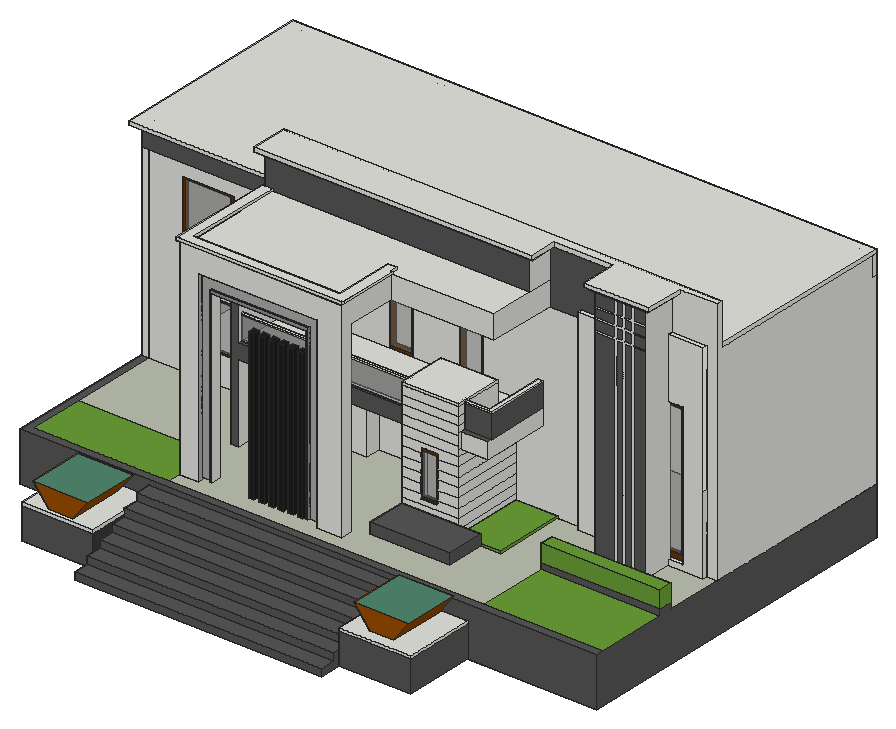
# SketchUp Ruby script. Lengths in inches.
U = 1.inch
M = Sketchup.active_model
def pt(a) = Geom::Point3d.new(a.map { |v| v * U })
def face(e, loops, mat)
  f = e.add_face(loops[0].map { |a| pt(a) })
  loops[1..].each { |l| e.add_face(l.map { |a| pt(a) }).erase! }
  f.material = f.back_material = mat if mat
  f
end
# faces: each face lists its corners as indices into pts; further lists are holes
def faces(e, pts, list, mat = nil) = list.each { |f| face(e, (f[0].is_a?(Array) ? f : [f]).map { |l| l.map { |i| pts[i] } }, mat) }
# xy, xz, yz: faces in a plane at the given z, y or x. An outline is a flat list of corners, or four numbers for a rectangle; further outlines are holes
def ring(l) = l.size == 4 ? [[l[0], l[1]], [l[2], l[1]], [l[2], l[3]], [l[0], l[3]]] : l.each_slice(2).to_a
def flat(e, list, mat, &to3) = list.each { |f| face(e, (f[0].is_a?(Array) ? f : [f]).map { |l| ring(l).map { |u, v| to3.(u, v) } }, mat) }
def xy(e, z, list, mat = nil) = flat(e, list, mat) { |x, y| [x, y, z] }
def xz(e, y, list, mat = nil) = flat(e, list, mat) { |x, z| [x, y, z] }
def yz(e, x, list, mat = nil) = flat(e, list, mat) { |y, z| [x, y, z] }
def lines(e, pts, list) = list.each { |a, b| e.add_line(pt(pts[a]), pt(pts[b])) }
# prism: a flat outline (further loops are holes) pulled along v
def prism(e, loops, v, mat = nil)
  f = face(e, loops, mat); d = Geom::Vector3d.new(v.map { |x| x * U })
  f.pushpull(f.normal.samedirection?(d) ? d.length : -d.length)
end
def box(e, o, s, mat = nil) = prism(e, [[o, [o[0] + s[0], o[1], o[2]], [o[0] + s[0], o[1] + s[1], o[2]], [o[0], o[1] + s[1], o[2]]]], [0, 0, s[2]], mat)
def at(x, y, z, deg = 0) = Geom::Transformation.translation(pt([x, y, z])) * Geom::Transformation.rotation(ORIGIN, Z_AXIS, deg.degrees)
def axes(o, x, y, z) = Geom::Transformation.new([*x, 0, *y, 0, *z, 0, *pt(o).to_a, 1])
def part(name) = M.definitions.add(name)
# library, detail: a bought-in or finely detailed component or shape, given as its bounding box
def library(name, o, s) = part(name).tap { |d| box(d.entities, o, s) }
def detail(e, o, s) = box(e.add_group.entities, o, s)
def put(e, d, t, mat = nil) = e.add_instance(d, t).tap { |i| i.material = mat if mat }
def group(e, t, mat = nil) = e.add_group.tap { |g| g.transformation = t; g.material = mat if mat }.entities
root = M.entities
M.materials.add("[Color C07]").color = [153, 76, 0]
M.materials.add("[Color C08]").color = [102, 51, 0]
M.materials.add("[Color M00]").color = [255, 255, 255]
M.materials.add("[Color M03]").color = [170, 170, 170]
M.materials.add("[Color M04]").color = [142, 142, 142]
M.materials.add("[Color M06]").color = [86, 86, 86]
M.materials.add("[Color M07]").color = [58, 58, 58]
M.materials.add("[Color M08]").color = [30, 30, 30]
M.materials.add("[Grass Dark Green]").color = [106, 157, 55]
M.materials.add("[Metal Seamed]").color = [118, 119, 115]
M.materials.add("[Pavers with Grass Brick]").color = [187, 192, 176]
M.materials.add("[Stone Vein Gray]").color = [166, 165, 165]
M.materials.add("[Translucent Glass Gray]").color = [128, 128, 128]
M.materials["[Translucent Glass Gray]"].alpha = 0.5
M.materials.add("[Vegetation Ivy Hedera]").color = [81, 134, 109]
M.materials.add("[Wood Veneer 01]").color = [120, 70, 37]
c1 = part("Group\#1")
xy(c1.entities,0,[[0,0,111.125,4.8125]])
xy(c1.entities,6.26,[[6.26,0,36.94,4.8125],[36.94,0,39.92,4.8125],[39.92,0,72.69,4.8125],[72.69,0,75.67,4.8125],[75.67,0,104.87,4.8125]],"[Color C08]")
xy(c1.entities,151.68,[[6.26,0,104.87,4.8125]],"[Color C08]")
xy(c1.entities,157.9375,[[0,0,111.125,4.8125]],"[Color C08]")
xz(c1.entities,0,[[[0,0,111.125,157.9375],[6.26,6.26,104.87,151.68]]],"[Color C08]")
xz(c1.entities,0,[[6.26,6.26,104.87,151.68]],"[Translucent Glass Gray]")
xz(c1.entities,4.8125,[[[0,0,111.125,157.9375],[6.26,6.26,104.87,151.68]]],"[Color C08]")
yz(c1.entities,0,[[0,0,4.8125,157.9375]],"[Color C08]")
yz(c1.entities,6.26,[[0,6.26,4.8125,151.68]],"[Color C08]")
yz(c1.entities,104.87,[[0,6.26,4.8125,151.68]],"[Color C08]")
yz(c1.entities,111.125,[[0,0,4.8125,157.9375]],"[Color C08]")
xy(root,-66.5625,[[11,144,11,684,900.0625,684,900.0625,144,209.9,144,209.9,145.85,99.84,145.85,99.84,144]])
xy(root,-66.5625,[[590.88,33.9375,700.95,144],[99.84,35.78,209.9,144],[99.84,144,209.9,145.85]],"[Color M06]")
xy(root,-18.5625,[[590.88,33.9375,700.95,144],[99.84,35.78,209.9,145.85]])
xy(root,-13.5625,[[[590.88,33.9375,700.95,144],[624.02,51.36,662.08,138.36]],[99.84,35.78,209.9,145.85],[624.02,51.36,662.08,138.36]])
xy(root,-9.6875,[[139.78,37.5,177.84,124.49]])
xy(root,6.25,[[719,386.8125,883.625,672]])
xy(root,9,[[501.4375,266.5625,589.01,342.0625],[589.01,266.5625,654.375,377.5625],[231.74,274.5625,231.74,351.0625,243.375,351.0625,243.375,386.8125,380.41,386.8125,380.41,351.0625,243.375,351.0625,243.375,274.5625],[501.4375,342.0625,501.4375,351.0625,478.41,351.0625,478.41,386.8125,883.625,386.8125,883.625,370.25,829.89,370.25,829.89,373.5,750.2,373.5,750.2,370.25,690.45,370.25,690.45,377.5625,589.01,377.5625,589.01,342.0625],[750.2,370.25,829.89,373.5],
  [11,377.5625,11,684,900.0625,684,900.0625,377.5625,883.625,377.5625,883.625,672,23,672,23,377.5625],[23,377.5625,231.74,386.8125],[23,386.8125,231.74,672]])
xy(root,9,[[11,144,900.0625,144,900.0625,156,23,156,23,377.5625,11,377.5625]],"[Color M06]")
xy(root,9,[[23,156,230.83,241.11],[716.24,156,900.0625,266.78]],"[Grass Dark Green]")
xy(root,9,[[[230.83,156,716.24,156,716.24,287.99,900.0625,287.99,900.0625,377.5625,883.625,377.5625,883.625,370.25,829.89,370.25,829.89,328,750.2,328,750.2,370.25,690.45,370.25,690.45,377.5625,654.375,377.5625,654.375,266.5625,624.0625,266.5625,624.0625,206.125,501.4375,206.125,501.4375,351.0625,478.41,351.0625,478.41,374.5625,380.41,374.5625,380.41,351.0625,243.375,351.0625,243.375,274.5625,231.74,274.5625,231.74,377.5625,23,377.5625,23,241.11,230.83,241.11],[442.4,176.6875,480.58,194.92],[331.03,183.97,339.78,194.35],[346.85,183.97,355.6,194.35],[362.1,183.97,370.85,194.35],[376.91,183.97,385.66,194.35],[391.66,183.97,400.41,194.35],[406.6,183.97,415.35,194.35]]],"[Pavers with Grass Brick]")
xy(root,9,[[501.4375,206.125,624.0625,266.5625]],"[Stone Vein Gray]")
xy(root,9.3125,[[231.74,176.6875,260.125,194.92]])
xy(root,12,[[589.01,266.5625,654.375,377.5625]],"[Grass Dark Green]")
xy(root,12.375,[[274.3,180,277.43,194.92],[260.125,183.375,274.3,194.92]])
xy(root,13.5625,[[422.47,180,425.53,194.92],[425.53,183.375,442.4,194.92]])
xy(root,17.02,[[599.9375,51.36,685.27,138.36]],"[Vegetation Ivy Hedera]")
xy(root,17.15,[[716.97,370.25,760.76,370.25,760.76,373.5,810.51,373.5,810.51,370.25,852.41,370.25,852.41,386.8125,716.97,386.8125],[760.76,370.25,810.51,373.5]])
xy(root,18,[[716.24,266.78,900.0625,287.99]])
xy(root,20.89,[[115.69,37.5,201.02,124.49]],"[Vegetation Ivy Hedera]")
xy(root,25.1875,[[501.4375,206.125,624.0625,266.5625]],"[Color M06]")
xy(root,42.92,[[532.43,266.5625,556.68,275.5625]])
xy(root,45,[[716.24,266.78,900.0625,287.99]],"[Grass Dark Green]")
xy(root,51.8,[[74.49,377.5625,153.11,386.8125]])
xy(root,110.3125,[[380.41,351.0625,478.41,374.5625],[380.41,374.5625,478.41,386.8125]])
xy(root,111.85,[[532.43,266.5625,556.68,275.5625]])
xy(root,127.36,[[74.49,377.5625,153.11,386.8125]])
xy(root,129,[[589.01,270.875,631.25,377.5625],[243.375,274.5625,501.4375,351.0625],[501.4375,342.0625,589.01,377.5625],[243.375,351.0625,283.875,377.5625],[283.875,351.0625,380.41,377.5625],
  [380.41,351.0625,478.41,377.5625],[478.41,351.0625,501.4375,377.5625],[380.41,377.5625,478.41,377.5625,478.41,386.8125,883.625,386.8125,883.625,672,243.375,672,243.375,386.8125,380.41,386.8125]])
xy(root,153,[[243.375,278.6875,501.4375,283.59],[589.01,278.6875,631.25,283.59],[243.375,283.59,501.4375,283.59,501.4375,342.0625,589.01,342.0625,589.01,283.59,623.4375,283.59,623.4375,377.5625,537.88,377.5625,537.88,386.8125,501.88,386.8125,501.88,377.5625,430.25,377.5625,430.25,386.8125,394.25,386.8125,394.25,377.5625,322.66,377.5625,322.66,386.8125,274.66,386.8125,274.66,377.5625,243.375,377.5625]])
xy(root,153,[[589.01,270.875,631.25,278.6875],[243.375,274.5625,501.4375,278.6875]],"[Color M06]")
xy(root,189,[[[501.4375,266.5625,589.01,342.0625],[504.68,269.8,585.77,338.82]],[504.68,269.8,585.77,338.82],[243.375,278.6875,501.4375,283.59],[589.01,278.6875,631.25,283.59],[623.4375,283.59,631.25,377.5625]])
xy(root,191,[[243.375,278.6875,501.4375,283.59],[589.01,278.6875,631.25,278.6875,631.25,377.5625,623.4375,377.5625,623.4375,283.59,589.01,283.59]])
xy(root,193,[[501.4375,266.5625,589.01,342.0625]])
xy(root,203.11,[[74.49,377.5625,153.11,386.8125]])
xy(root,236.29,[[716.97,370.25,716.97,386.8125,852.41,386.8125,852.41,370.25,810.51,370.25,810.51,373.5,760.76,373.5,760.76,370.25],[760.76,370.25,810.51,373.5]])
xy(root,237,[[274.66,377.5625,322.66,386.8125],[394.25,377.5625,430.25,386.8125],[501.88,377.5625,537.88,386.8125]])
xy(root,238.5,[[331.03,183.97,339.78,194.35],[346.85,183.97,355.6,194.35],[362.1,183.97,370.85,194.35],[376.91,183.97,385.66,194.35],[391.66,183.97,400.41,194.35],
  [406.6,183.97,415.35,194.35]],"[Color M08]")
xy(root,246.62,[[750.2,370.25,829.89,373.5]])
xy(root,273.9375,[[277.43,180,422.47,194.92],[274.3,183.375,277.43,194.92],[422.47,183.375,425.53,194.92]])
xy(root,277.9375,[[277.43,183.375,422.47,194.92]])
xy(root,277.9375,[[274.3,180,425.53,183.375]],"[Color M04]")
xy(root,278.67,[[74.49,377.5625,153.11,386.8125]])
xy(root,293.9375,[[272.1,206.49,272.1,377.5625,615.91,377.5625,615.91,293.74,464.91,293.74,464.91,206.49,435.8,206.49,435.8,293.74,430.51,302.06,423.89,309.35,416.12,315.42,407.43,320.07,398.08,323.17,388.33,324.64,378.48,324.43,368.81,322.54,359.6,319.04,351.12,314.02,343.61,307.625,337.31,300.05,337.31,206.49]])
xy(root,297.1875,[[260.125,183.375,393.59,183.375,260.125,193.64],[393.59,183.375,442.4,183.375,442.4,194.92,260.125,194.92,260.125,193.64],[260.125,193.64,260.125,194.92,243.375,194.92],[231.74,194.92,243.375,274.5625],[243.375,194.92,243.375,377.5625,272.1,377.5625,272.1,206.49,464.91,206.49,464.91,293.74,615.91,293.74,615.91,377.5625,640.81,377.5625,640.81,270.875,480.58,270.875,480.58,194.92],
  [337.31,206.49,337.31,300.05,343.61,307.625,351.12,314.02,359.6,319.04,368.81,322.54,378.48,324.43,388.33,324.64,398.08,323.17,407.43,320.07,416.12,315.42,423.89,309.35,430.51,302.06,435.8,293.74,435.8,206.49],[243.375,377.5625,480.76,386.8125],[11,676.625,900.0625,684]])
xy(root,297.1875,[[260.125,176.6875,442.4,176.6875,442.4,179.62,393.59,183.375,260.125,183.375],[442.4,179.62,442.4,183.375,393.59,183.375]],"[Color M03]")
xy(root,309.625,[[690.45,370.25,750.2,377.5625]])
xy(root,327.1875,[[0,367.4375,0,684,11,684,11,676.625,900.0625,676.625,900.0625,386.8125,231.74,386.8125,231.74,367.4375],[11,676.625,900.0625,684]])
xy(root,328.1875,[[829.89,370.25,883.625,377.5625]])
xy(root,333.1875,[[227.99,173.625,228.81,176.6875],[228.81,173.625,231.74,176.6875],[231.74,173.625,480.58,176.6875],[480.58,173.625,483.95,176.6875],[227.99,176.6875,231.74,340.0625],
  [231.74,176.6875,231.74,340.0625,243.375,340.0625,243.375,189.17,318.2,189.17,480.58,176.6875],[480.58,176.6875,318.2,189.17,467.72,189.17,467.72,282.5,480.58,282.5],[480.58,176.6875,483.95,270.875],[243.375,189.17,318.2,189.17,243.375,194.92],[318.2,189.17,467.72,189.17,467.72,282.5,480.58,282.5,480.58,270.875,640.81,270.875,640.81,340.0625,243.375,340.0625,243.375,194.92],
  [231.74,340.0625,640.81,386.8125],[0,367.4375,231.74,367.4375,231.74,386.8125,900.0625,386.8125,900.0625,684,0,684]])
xy(root,337.1875,[[227.99,173.625,483.95,173.625,483.95,270.875,480.58,270.875,480.58,282.5,467.72,282.5,467.72,189.17,243.375,189.17,243.375,340.0625,227.99,340.0625]])
xy(root,381.1875,[[746.76,321.5,746.76,377.5625,750.2,377.5625,750.2,328,829.89,328,829.89,377.5625,836.7,377.5625,836.7,321.5],[750.2,328,829.89,377.5625],[230.37,336.3125,647.56,340.0625],[230.37,340.0625,231.74,386.8125],[640.81,340.0625,647.56,377.5625]])
xy(root,385.1875,[[741.39,318.9375,741.39,373.6875,746.76,373.6875,746.76,321.5,836.7,321.5,836.7,377.5625,841.57,377.5625,841.57,318.9375],[222.81,330.5,647.56,336.3125],[647.56,330.5,651.06,373.6875],[222.81,336.3125,230.37,386.8125],[647.56,373.6875,746.76,377.5625],
  [746.76,373.6875,750.2,377.5625]])
xy(root,391.1875,[[741.39,318.9375,841.57,318.9375,841.57,377.5625,900.0625,377.5625,900.0625,386.8125,222.81,386.8125,222.81,330.5,651.06,330.5,651.06,373.6875,741.39,373.6875]])
xz(root,33.9375,[[590.88,-18.5625,700.95,-13.5625]])
xz(root,33.9375,[[590.88,-66.5625,700.95,-18.5625]],"[Color M06]")
xz(root,35.78,[[99.84,-18.5625,209.9,-13.5625]])
xz(root,35.78,[[99.84,-66.5625,209.9,-18.5625]],"[Color M06]")
xz(root,37.5,[[139.78,-9.6875,177.84,-9.6875,201.02,20.89,115.69,20.89]],"[Color C07]")
xz(root,51.36,[[624.02,-13.5625,662.08,-13.5625,685.27,17.02,599.9375,17.02]],"[Color C07]")
xz(root,124.49,[[139.78,-9.6875,115.69,20.89,201.02,20.89,177.84,-9.6875]],"[Color C07]")
xz(root,138.36,[[624.02,-13.5625,599.9375,17.02,685.27,17.02,662.08,-13.5625]],"[Color C07]")
xz(root,144,[[590.88,-66.5625,700.95,-18.5625],[590.88,-18.5625,700.95,-13.5625]])
xz(root,144,[[11,-66.5625,590.88,-66.5625,590.88,-13.5625,700.95,-13.5625,700.95,-66.5625,900.0625,-66.5625,900.0625,9,11,9],[590.88,-18.5625,700.95,-13.5625]],"[Color M06]")
xz(root,145.85,[[99.84,-66.5625,209.9,-18.5625],[99.84,-18.5625,209.9,-13.5625]])
xz(root,173.625,[[227.99,333.1875,483.95,337.1875]])
xz(root,176.6875,[[442.4,9,480.58,9,480.58,333.1875,231.74,333.1875,231.74,9.3125,260.125,9.3125,260.125,297.1875,442.4,297.1875]])
xz(root,180,[[274.3,12.375,277.43,12.375,277.43,273.9375,422.47,273.9375,422.47,13.5625,425.53,13.5625,425.53,277.9375,274.3,277.9375]],"[Color M04]")
xz(root,183.375,[[274.3,273.9375,277.43,277.9375],[422.47,273.9375,425.53,277.9375]])
xz(root,183.375,[[260.125,12.375,274.3,12.375,274.3,277.9375,425.53,277.9375,425.53,13.5625,442.4,13.5625,442.4,297.1875,260.125,297.1875]],"[Color M03]")
xz(root,183.97,[[331.03,9,339.78,238.5],[346.85,9,355.6,238.5],[362.1,9,370.85,238.5],[376.91,9,385.66,238.5],[391.66,9,400.41,238.5],
  [406.6,9,415.35,238.5]],"[Color M08]")
xz(root,189.17,[[243.375,333.1875,467.72,337.1875]])
xz(root,194.35,[[331.03,9,339.78,238.5],[346.85,9,355.6,238.5],[362.1,9,370.85,238.5],[376.91,9,385.66,238.5],[391.66,9,400.41,238.5],
  [406.6,9,415.35,238.5]],"[Color M08]")
xz(root,194.92,[[442.4,9,480.58,297.1875],[231.74,9.3125,260.125,297.1875],[260.125,12.375,260.125,297.1875,442.4,297.1875,442.4,13.5625,425.53,13.5625,425.53,273.9375,422.47,273.9375,422.47,277.9375,277.43,277.9375,277.43,273.9375,274.3,273.9375,274.3,12.375],[274.3,12.375,277.43,273.9375],[422.47,13.5625,425.53,273.9375],
  [277.43,273.9375,422.47,277.9375]])
xz(root,206.125,[[501.4375,9,624.0625,25.1875]],"[Color M06]")
xz(root,206.49,[[272.1,293.9375,337.31,297.1875],[435.8,293.9375,464.91,297.1875]])
xz(root,266.5625,[[501.4375,9,589.01,19.37],[501.4375,19.37,589.01,25.1875],[501.4375,25.1875,589.01,33.68],[501.4375,33.68,589.01,33.68,589.01,47.99,558.02,47.99,558.02,41.57,531.09,41.57,531.09,47.99,501.4375,47.99],[[531.09,41.57,558.02,113.19],[532.43,42.92,556.68,111.85]],
  [501.4375,47.99,531.09,62.3],[558.02,47.99,589.01,62.3],[501.4375,62.3,531.09,76.62],[558.02,62.3,589.01,76.62],[501.4375,76.62,531.09,90.93],
  [558.02,76.62,589.01,90.93],[501.4375,90.93,531.09,105.24],[558.02,90.93,589.01,105.24],[501.4375,105.24,531.09,105.24,531.09,113.19,558.02,113.19,558.02,105.24,589.01,105.24,589.01,119.55,501.4375,119.55],[501.4375,119.55,589.01,133.87],
  [501.4375,133.87,589.01,148.18],[501.4375,148.18,589.01,162.49],[501.4375,162.49,589.01,174.81],[501.4375,174.81,589.01,189],[501.4375,189,589.01,193]])
xz(root,266.5625,[[589.01,9,624.0625,12],[589.01,12,624.0625,25.1875]],"[Color M06]")
xz(root,266.5625,[[624.0625,9,654.375,12]],"[Grass Dark Green]")
xz(root,266.78,[[716.24,9,900.0625,18]],"[Color M06]")
xz(root,266.78,[[716.24,18,900.0625,45]],"[Grass Dark Green]")
xz(root,270.875,[[589.01,129,631.25,153],[480.58,297.1875,640.81,333.1875],[480.58,333.1875,483.95,337.1875]])
xz(root,274.5625,[[231.74,9,243.375,9,243.375,129,501.4375,129,501.4375,153,243.375,153,243.375,297.1875,231.74,297.1875]],"[Color M06]")
xz(root,275.5625,[[532.43,42.92,556.68,111.85]])
xz(root,278.6875,[[243.375,189,501.4375,191],[589.01,189,631.25,191]])
xz(root,278.6875,[[589.01,153,631.25,189]],"[Color M06]")
xz(root,278.6875,[[243.375,153,501.4375,189]],"[Translucent Glass Gray]")
xz(root,282.5,[[467.72,333.1875,480.58,337.1875]])
xz(root,283.59,[[589.01,153,623.4375,189],[243.375,189,501.4375,191],[589.01,189,623.4375,191]])
xz(root,283.59,[[243.375,153,501.4375,189]],"[Translucent Glass Gray]")
xz(root,287.99,[[716.24,9,900.0625,18]],"[Color M06]")
xz(root,287.99,[[716.24,18,900.0625,45]],"[Grass Dark Green]")
xz(root,293.74,[[464.91,293.9375,615.91,297.1875]])
xz(root,318.9375,[[741.39,385.1875,841.57,391.1875]])
xz(root,321.5,[[746.76,381.1875,836.7,385.1875]])
xz(root,328,[[[781.13,9,784.6,9,784.6,321.8,793.32,321.8,793.32,9,796.79,9,796.79,321.8,806.82,321.8,806.82,9,810.29,9,810.29,321.8,829.89,321.8,829.89,324.21,810.29,324.21,810.29,339.86,829.89,339.86,829.89,342.27,810.29,342.27,810.29,355.8,829.89,355.8,829.89,358.21,810.29,358.21,810.29,381.1875,806.82,381.1875,806.82,358.21,796.79,358.21,796.79,381.1875,793.32,381.1875,793.32,358.21,784.6,358.21,784.6,381.1875,781.13,381.1875,781.13,358.21,750.2,358.21,750.2,355.8,781.13,355.8,781.13,342.27,750.2,342.27,750.2,339.86,781.13,339.86,781.13,324.21,750.2,324.21,750.2,321.8,781.13,321.8],[796.79,324.21,806.82,339.86],[784.6,324.21,793.32,339.86],[796.79,342.27,806.82,355.8],[784.6,342.27,793.32,355.8]]])
xz(root,328,[[750.2,9,781.13,321.8],[784.6,9,793.32,321.8],[796.79,9,806.82,321.8],[810.29,9,829.89,321.8],[750.2,324.21,781.13,339.86],
  [784.6,324.21,793.32,339.86],[796.79,324.21,806.82,339.86],[810.29,324.21,829.89,339.86],[750.2,342.27,781.13,355.8],[784.6,342.27,793.32,355.8],
  [796.79,342.27,806.82,355.8],[810.29,342.27,829.89,355.8],[750.2,358.21,781.13,381.1875],[784.6,358.21,793.32,381.1875],[796.79,358.21,806.82,381.1875],
  [810.29,358.21,829.89,381.1875]],"[Color M06]")
xz(root,330.5,[[222.81,385.1875,651.06,391.1875]])
xz(root,336.3125,[[230.37,381.1875,647.56,385.1875]])
xz(root,340.0625,[[227.99,333.1875,231.74,337.1875],[231.74,333.1875,243.375,337.1875]])
xz(root,340.0625,[[243.375,333.1875,640.81,333.1875,640.81,381.1875,231.74,381.1875,231.74,337.1875,243.375,337.1875]],"[Color M06]")
xz(root,342.0625,[[501.4375,129,589.01,153],[501.4375,153,589.01,189],[501.4375,189,589.01,193]])
xz(root,351.0625,[[243.375,9,380.41,9,380.41,110.3125,478.41,110.3125,478.41,9,501.4375,9,501.4375,129,243.375,129]])
xz(root,367.4375,[[0,327.1875,231.74,333.1875]])
xz(root,370.25,[[[690.45,9,883.625,9,883.625,328.1875,829.89,328.1875,829.89,246.62,750.2,246.62,750.2,309.625,690.45,309.625],[716.97,17.15,852.41,236.29]]])
xz(root,373.5,[[750.2,9,829.89,17.15],[750.2,17.15,829.89,236.29],[750.2,236.29,829.89,246.62]])
xz(root,373.6875,[[651.06,385.1875,741.39,391.1875]])
xz(root,374.5625,[[380.41,9,478.41,110.3125]])
xz(root,377.5625,[[11,9,23,297.1875],[[23,9,231.74,297.1875],[74.49,203.11,153.11,278.67],[74.49,51.8,153.11,127.36]],[654.375,9,690.45,9,690.45,297.1875,615.91,297.1875,615.91,293.9375,272.1,293.9375,272.1,297.1875,243.375,297.1875,243.375,153,274.66,153,274.66,237,322.66,237,322.66,153,394.25,153,394.25,237,430.25,237,430.25,153,501.88,153,501.88,237,537.88,237,537.88,153,623.4375,153,623.4375,191,631.25,191,631.25,129,589.01,129,589.01,12,654.375,12],[589.01,9,654.375,12],[883.625,9,900.0625,9,900.0625,391.1875,841.57,391.1875,841.57,385.1875,836.7,385.1875,836.7,381.1875,829.89,381.1875,829.89,328.1875,883.625,328.1875],
  [272.1,293.9375,480.76,297.1875],[750.2,297.1875,829.89,381.1875]])
xz(root,377.5625,[[11,297.1875,231.74,327.82],[640.81,297.1875,690.45,297.1875,690.45,309.625,750.2,309.625,750.2,381.1875,746.76,381.1875,746.76,385.1875,647.56,385.1875,647.56,381.1875,640.81,381.1875]],"[Color M06]")
xz(root,386.8125,[[243.375,9,380.41,129],[478.41,9,478.41,129,716.97,129,716.97,17.15,719,17.15,719,9],[719,9,719,17.15,852.41,17.15,852.41,129,883.625,129,883.625,9],[716.97,17.15,719,129],[719,17.15,852.41,129],
  [[380.41,110.3125,380.41,129,243.375,129,243.375,297.1875,883.625,297.1875,883.625,129,852.41,129,852.41,236.29,716.97,236.29,716.97,129,478.41,129,478.41,110.3125],[274.66,153,322.66,237],[394.25,153,430.25,237],[501.88,153,537.88,237]],[243.375,297.1875,883.625,327.1875],[231.74,327.1875,243.375,333.1875],[243.375,327.1875,640.81,333.1875],[640.81,327.1875,883.625,333.1875],
  [883.625,327.1875,900.0625,333.1875],[231.74,333.1875,243.375,381.1875],[243.375,333.1875,640.81,381.1875],[640.81,333.1875,900.0625,391.1875],[230.37,381.1875,243.375,385.1875],
  [243.375,381.1875,640.81,385.1875],[222.81,385.1875,243.375,391.1875],[243.375,385.1875,640.81,391.1875]])
xz(root,672,[[719,6.25,883.625,9],[23,9,231.74,297.1875],[231.74,9,243.375,129],[243.375,9,719,129],[719,9,883.625,129],
  [231.74,129,243.375,297.1875],[243.375,129,883.625,297.1875]])
xz(root,684,[[11,9,900.0625,297.1875],[11,297.1875,900.0625,327.1875],[0,327.1875,11,327.82],[11,327.1875,11,327.82,0,327.82,0,333.1875,900.0625,333.1875,900.0625,327.1875]])
xz(root,684,[[11,-66.5625,900.0625,9]],"[Color M06]")
yz(root,0,[[367.4375,327.1875,684,327.82],[367.4375,327.82,684,333.1875]])
yz(root,11,[[377.5625,9,684,297.1875],[377.5625,297.1875,684,327.82]])
yz(root,11,[[144,-66.5625,684,9]],"[Color M06]")
yz(root,23,[[377.5625,9,386.8125,129],[386.8125,9,672,297.1875],[377.5625,129,386.8125,297.1875]])
yz(root,74.49,[[377.5625,51.8,386.8125,127.36],[377.5625,203.11,386.8125,278.67]])
yz(root,99.84,[[35.78,-18.5625,145.85,-13.5625]])
yz(root,99.84,[[35.78,-66.5625,145.85,-18.5625]],"[Color M06]")
yz(root,153.11,[[377.5625,51.8,386.8125,127.36],[377.5625,203.11,386.8125,278.67]])
yz(root,209.9,[[35.78,-18.5625,145.85,-13.5625]])
yz(root,209.9,[[35.78,-66.5625,145.85,-18.5625]],"[Color M07]")
yz(root,222.81,[[330.5,385.1875,386.8125,391.1875]])
yz(root,227.99,[[173.625,333.1875,340.0625,337.1875]])
yz(root,230.37,[[336.3125,381.1875,386.8125,385.1875]])
yz(root,231.74,[[274.5625,9,377.5625,297.1875],[386.8125,9,672,129],[176.6875,9.3125,176.6875,333.1875,367.4375,333.1875,367.4375,327.1875,377.5625,327.1875,377.5625,297.1875,194.92,297.1875,194.92,9.3125],[377.5625,129,386.8125,297.1875],[377.5625,297.1875,386.8125,327.1875],
  [367.4375,327.1875,377.5625,327.82],[377.5625,327.1875,386.8125,327.1875,386.8125,333.1875,367.4375,333.1875,367.4375,327.82,377.5625,327.82],[340.0625,333.1875,386.8125,381.1875]])
yz(root,243.375,[[274.5625,9,351.0625,129],[377.5625,129,386.8125,177.1875],[274.5625,153,278.6875,153,278.6875,191,283.59,191,283.59,153,377.5625,153,377.5625,297.1875,274.5625,297.1875],[377.5625,177.1875,386.8125,297.1875],[278.6875,189,283.59,191],
  [189.17,297.1875,194.92,333.1875],[194.92,297.1875,277.27,333.1875],[189.17,333.1875,340.0625,337.1875]])
yz(root,260.125,[[183.375,12.375,194.92,297.1875]])
yz(root,260.125,[[176.6875,9.3125,194.92,9.3125,194.92,12.375,183.375,12.375,183.375,297.1875,176.6875,297.1875]],"[Color M03]")
yz(root,272.1,[[206.49,293.9375,353.55,297.1875],[353.55,293.9375,377.5625,297.1875]])
yz(root,274.3,[[183.375,12.375,194.92,273.9375]])
yz(root,274.3,[[180,12.375,183.375,277.9375]],"[Color M04]")
yz(root,274.66,[[377.5625,153,386.8125,237]])
yz(root,277.43,[[180,12.375,194.92,273.9375],[183.375,273.9375,194.92,277.9375]])
yz(root,322.66,[[377.5625,153,386.8125,237]])
yz(root,331.03,[[183.97,9,194.35,238.5]],"[Color M08]")
yz(root,337.31,[[206.49,293.9375,300.05,297.1875]])
yz(root,339.78,[[183.97,9,194.35,238.5]],"[Color M08]")
yz(root,346.85,[[183.97,9,194.35,238.5]],"[Color M08]")
yz(root,355.6,[[183.97,9,194.35,238.5]],"[Color M08]")
yz(root,362.1,[[183.97,9,194.35,238.5]],"[Color M08]")
yz(root,370.85,[[183.97,9,194.35,238.5]],"[Color M08]")
yz(root,376.91,[[183.97,9,194.35,238.5]],"[Color M08]")
yz(root,380.41,[[351.0625,9,374.5625,110.3125],[374.5625,9,386.8125,110.3125]])
yz(root,385.66,[[183.97,9,194.35,238.5]],"[Color M08]")
yz(root,391.66,[[183.97,9,194.35,238.5]],"[Color M08]")
yz(root,394.25,[[377.5625,153,386.8125,237]])
yz(root,400.41,[[183.97,9,194.35,238.5]],"[Color M08]")
yz(root,406.6,[[183.97,9,194.35,238.5]],"[Color M08]")
yz(root,415.35,[[183.97,9,194.35,238.5]],"[Color M08]")
yz(root,422.47,[[180,13.5625,194.92,273.9375],[183.375,273.9375,194.92,277.9375]])
yz(root,425.53,[[183.375,13.5625,194.92,273.9375]])
yz(root,425.53,[[180,13.5625,183.375,277.9375]],"[Color M04]")
yz(root,430.25,[[377.5625,153,386.8125,237]])
yz(root,435.8,[[206.49,293.9375,293.74,297.1875]])
yz(root,442.4,[[183.375,13.5625,194.92,297.1875]])
yz(root,442.4,[[176.6875,9,176.6875,297.1875,183.375,297.1875,183.375,13.5625,194.92,13.5625,194.92,9]],"[Color M03]")
yz(root,464.91,[[206.49,293.9375,293.74,297.1875]])
yz(root,467.72,[[189.17,333.1875,282.5,337.1875]])
yz(root,478.41,[[351.0625,9,374.5625,110.3125],[374.5625,9,386.8125,110.3125]])
yz(root,480.58,[[176.6875,9,194.92,9,194.92,297.1875,270.875,297.1875,270.875,333.1875,176.6875,333.1875],[270.875,333.1875,282.5,337.1875]])
yz(root,483.95,[[173.625,333.1875,176.6875,337.1875],[176.6875,333.1875,270.875,337.1875]])
yz(root,501.4375,[[266.5625,9,351.0625,19.37],[266.5625,19.37,351.0625,33.68],[266.5625,33.68,351.0625,47.99],[266.5625,47.99,351.0625,62.3],[266.5625,62.3,351.0625,76.62],
  [266.5625,76.62,351.0625,90.93],[266.5625,90.93,351.0625,105.24],[266.5625,105.24,351.0625,119.55],[266.5625,119.55,351.0625,129],[266.5625,129,274.5625,153],
  [274.5625,129,342.0625,153],[266.5625,153,278.6875,162.49],[278.6875,153,283.59,189],[283.59,153,342.0625,189],[266.5625,162.49,278.6875,174.81],
  [266.5625,174.81,278.6875,189],[266.5625,189,278.6875,193],[278.6875,189,283.59,191],[283.59,189,342.0625,193],[278.6875,191,283.59,193]])
yz(root,501.4375,[[206.125,9,266.5625,25.1875]],"[Color M06]")
yz(root,501.88,[[377.5625,153,386.8125,237]])
yz(root,532.43,[[266.5625,42.92,275.5625,111.85]])
yz(root,537.88,[[377.5625,153,386.8125,237]])
yz(root,556.68,[[266.5625,42.92,275.5625,111.85]])
yz(root,589.01,[[266.5625,9,377.5625,12],[266.5625,12,377.5625,19.37],[266.5625,19.37,377.5625,33.68],[266.5625,33.68,377.5625,47.99],[266.5625,47.99,377.5625,62.3],
  [266.5625,62.3,377.5625,76.62],[266.5625,76.62,377.5625,90.93],[266.5625,90.93,377.5625,105.24],[266.5625,105.24,377.5625,119.55],[266.5625,119.55,377.5625,129],
  [266.5625,129,270.875,153],[270.875,129,342.0625,153],[266.5625,153,278.6875,162.49],[278.6875,153,283.59,189],[283.59,153,342.0625,189],
  [266.5625,162.49,278.6875,174.81],[266.5625,174.81,278.6875,189],[266.5625,189,278.6875,193],[278.6875,189,283.59,191],[283.59,189,342.0625,193],
  [278.6875,191,283.59,193]])
yz(root,590.88,[[33.9375,-18.5625,144,-13.5625]])
yz(root,590.88,[[33.9375,-66.5625,144,-18.5625]],"[Color M07]")
yz(root,615.91,[[293.74,293.9375,377.5625,297.1875]])
yz(root,623.4375,[[283.59,153,377.5625,189],[283.59,189,377.5625,191]])
yz(root,624.0625,[[206.125,9,266.5625,25.1875]],"[Color M06]")
yz(root,631.25,[[270.875,129,377.5625,153],[278.6875,189,377.5625,191]])
yz(root,631.25,[[278.6875,153,377.5625,189]],"[Color M06]")
yz(root,640.81,[[270.875,297.1875,377.5625,333.1875],[340.0625,333.1875,377.5625,381.1875]])
yz(root,647.56,[[336.3125,381.1875,377.5625,385.1875]])
yz(root,651.06,[[330.5,385.1875,373.6875,391.1875]])
yz(root,654.375,[[266.5625,9,377.5625,12]],"[Grass Dark Green]")
yz(root,690.45,[[370.25,9,377.5625,309.625]])
yz(root,700.95,[[33.9375,-18.5625,144,-13.5625]])
yz(root,700.95,[[33.9375,-66.5625,144,-18.5625]],"[Color M06]")
yz(root,716.24,[[266.78,9,287.99,18]],"[Color M06]")
yz(root,716.24,[[266.78,18,287.99,45]],"[Grass Dark Green]")
yz(root,716.97,[[370.25,17.15,386.8125,236.29]])
yz(root,741.39,[[318.9375,385.1875,373.6875,391.1875]])
yz(root,746.76,[[321.5,381.1875,377.5625,385.1875]])
yz(root,750.2,[[328,9,328,381.1875,377.5625,381.1875,377.5625,309.625,370.25,309.625,370.25,246.62,373.5,246.62,373.5,9],[370.25,297.1875,377.5625,309.625]])
yz(root,829.89,[[328,9,373.5,9,373.5,246.62,370.25,246.62,370.25,328.1875,377.5625,328.1875,377.5625,381.1875,328,381.1875],[370.25,297.1875,377.5625,328.1875]])
yz(root,836.7,[[321.5,381.1875,377.5625,385.1875]])
yz(root,841.57,[[318.9375,385.1875,377.5625,391.1875]])
yz(root,852.41,[[370.25,17.15,386.8125,236.29]])
yz(root,883.625,[[386.8125,6.25,672,9],[370.25,9,377.5625,129],[377.5625,9,386.8125,297.1875],[386.8125,9,672,129],[386.8125,129,672,297.1875]])
yz(root,883.625,[[370.25,129,377.5625,328.1875]],"[Color M00]")
yz(root,900.0625,[[377.5625,9,684,9,684,297.1875,676.625,297.1875,676.625,327.1875,386.8125,327.1875,386.8125,391.1875,377.5625,391.1875],[676.625,297.1875,684,327.1875],[386.8125,327.1875,684,333.1875]])
yz(root,900.0625,[[144,-66.5625,684,-66.5625,684,9,287.99,9,287.99,18,266.78,18,266.78,9,144,9]],"[Color M06]")
yz(root,900.0625,[[266.78,18,287.99,45]],"[Grass Dark Green]")
p = [[624.02,51.36,-13.5625],[599.9375,51.36,17.02],[599.9375,138.36,17.02],[624.02,138.36,-13.5625],[685.27,51.36,17.02],[662.08,51.36,-13.5625],
  [662.08,138.36,-13.5625],[685.27,138.36,17.02],[139.78,37.5,-9.6875],[115.69,37.5,20.89],[115.69,124.49,20.89],[139.78,124.49,-9.6875],
  [201.02,37.5,20.89],[177.84,37.5,-9.6875],[177.84,124.49,-9.6875],[201.02,124.49,20.89],[435.8,293.74,297.1875],[430.51,302.06,297.1875],
  [430.51,302.06,293.9375],[435.8,293.74,293.9375],[343.61,307.625,297.1875],[337.31,300.05,297.1875],[337.31,300.05,293.9375],[343.61,307.625,293.9375],
  [423.89,309.35,297.1875],[423.89,309.35,293.9375],[351.12,314.02,297.1875],[351.12,314.02,293.9375],[416.12,315.42,297.1875],[416.12,315.42,293.9375],
  [359.6,319.04,297.1875],[359.6,319.04,293.9375],[407.43,320.07,297.1875],[407.43,320.07,293.9375],[368.81,322.54,297.1875],[368.81,322.54,293.9375],
  [398.08,323.17,297.1875],[398.08,323.17,293.9375],[378.48,324.43,297.1875],[378.48,324.43,293.9375],[388.33,324.64,297.1875],[388.33,324.64,293.9375],
  [480.58,176.6875,333.1875],[318.2,189.17,333.1875],[243.375,194.92,333.1875],[243.375,194.92,297.1875],[260.125,193.64,297.1875],[393.59,183.375,297.1875],
  [442.4,179.62,297.1875],[480.54,176.69,297.1875],[480.58,176.6875,297.1875],[-687.36,-1089.39,13.32],[-686.18,-1089.39,13.32],[-521.02,-1130.43,297.1875],
  [-521.02,-1130.43,333.1875],[-491.46,-1589.17,-21.0625],[-673.46,-1589.17,-21.0625],[-491.46,-1613.17,-32.4375],[-673.46,-1613.17,-32.4375],[-491.46,-1661.17,-55.1875],
  [-673.46,-1661.17,-55.1875],[585.77,278.6875,189],[585.77,278.6875,193],[585.77,269.8,189],[585.77,269.8,193],[504.68,338.82,189],
  [504.68,338.82,193],[585.77,283.59,189],[585.77,283.59,193],[504.68,283.59,189],[504.68,283.59,193],[504.68,278.6875,189],
  [504.68,278.6875,193],[504.68,269.8,189],[504.68,269.8,193],[585.77,338.82,189],[585.77,338.82,193],[272.1,377.5625,297.1875],
  [272.1,380.99,297.1875],[231.74,672,297.1875],[231.74,672,333.1875],[23,672,297.1875],[23,672,333.1875],[23,386.8125,297.1875],
  [23,386.8125,333.1875],[243.375,672,297.1875],[243.375,672,333.1875],[883.625,672,297.1875],[883.625,672,333.1875],[719,386.8125,9],
  [719,386.8125,6.25],[480.54,176.6875,297.1875],[231.74,176.6875,333.1875],[231.74,176.6875,337.1875],[480.58,176.6875,337.1875],[229.28,684,327.82],
  [228.81,684,327.82]]
faces(root,p,[[0,1,2,3],[4,5,6,7],[8,9,10,11],[12,13,14,15]],"[Color C07]")
faces(root,p,[[16,17,18,19],[20,21,22,23],[17,24,25,18],[26,20,23,27],[24,28,29,25],[30,26,27,31],[28,32,33,29],[34,30,31,35],
  [32,36,37,33],[38,34,35,39],[36,40,41,37],[40,38,39,41],[42,43,44,45,46,47,48,49,50]])
lines(root,p,[[51,52],[53,54],[55,56],[57,58],[59,60],[61,62],[63,64],[65,66],[67,68],[69,70],[71,72],[73,74],
  [75,76],[77,78],[79,80],[81,82],[83,84],[85,86],[87,88],[89,90],[91,49],[92,93],[42,94],[95,80],
  [96,95]])
g1 = group(root,at(274.66,377.5625,153))
xy(g1,0,[[0,1.5,48,9.125]])
xy(g1,4.9,[[4.9,1.5,43.1,3.125],[4.9,3.125,43.1,9.125]],"[Wood Veneer 01]")
xy(g1,34.09,[[9.11,0,20.42,1.625],[9.11,1.625,10.67,2]],"[Metal Seamed]")
xy(g1,37.09,[[10.67,0,20.42,1.625]],"[Metal Seamed]")
xy(g1,38.72,[[9.11,0,10.67,2]],"[Metal Seamed]")
xy(g1,79.1,[[4.9,1.5,43.1,3.125]])
xy(g1,79.1,[[4.9,3.125,43.1,9.125]],"[Wood Veneer 01]")
xy(g1,84,[[0,1.5,48,9.125]],"[Wood Veneer 01]")
xz(g1,0,[[9.11,34.09,20.42,34.09,20.42,37.09,10.67,37.09,10.67,38.72,9.11,38.72]],"[Metal Seamed]")
xz(g1,1.5,[[[0,0,48,84],[4.9,4.9,43.1,79.1]]],"[Wood Veneer 01]")
xz(g1,1.625,[[10.67,34.09,20.42,37.09]],"[Wood Veneer 01]")
xz(g1,2,[[[9.83,33.47,10.6,33.55,11.3125,33.83,11.93,34.28,12.41,34.875,12.72,35.57,12.84,36.33,12.76,37.09,12.49,37.81,12.03,38.43,11.4375,38.91,10.74,39.22,9.98,39.34,9.22,39.26,8.5,38.98,7.88,38.53,7.4,37.9375,7.09,37.23,6.97,36.48,7.05,35.71,7.33,35,7.78,34.38,8.375,33.9,9.08,33.59],[9.11,34.09,10.67,38.72]]],"[Metal Seamed]")
xz(g1,3.125,[[9.83,33.47,10.6,33.55,11.3125,33.83,11.93,34.28,12.41,34.875,12.72,35.57,12.84,36.33,12.76,37.09,12.49,37.81,12.03,38.43,11.4375,38.91,10.74,39.22,9.98,39.34,9.22,39.26,8.5,38.98,7.88,38.53,7.4,37.9375,7.09,37.23,6.97,36.48,7.05,35.71,7.33,35,7.78,34.38,8.375,33.9,9.08,33.59]])
xz(g1,3.125,[[[4.9,4.9,43.1,79.1],[9.83,33.47,9.08,33.59,8.375,33.9,7.78,34.38,7.33,35,7.05,35.71,6.97,36.48,7.09,37.23,7.4,37.9375,7.88,38.53,8.5,38.98,9.22,39.26,9.98,39.34,10.74,39.22,11.4375,38.91,12.03,38.43,12.49,37.81,12.76,37.09,12.84,36.33,12.72,35.57,12.41,34.875,11.93,34.28,11.3125,33.83,10.6,33.55]]],"[Wood Veneer 01]")
xz(g1,9.125,[[[0,0,48,84],[4.9,4.9,43.1,79.1]]],"[Wood Veneer 01]")
yz(g1,0,[[1.5,0,9.125,84]],"[Wood Veneer 01]")
yz(g1,4.9,[[1.5,4.9,3.125,79.1],[3.125,4.9,9.125,79.1]],"[Wood Veneer 01]")
yz(g1,9.11,[[0,34.09,2,38.72]],"[Metal Seamed]")
yz(g1,10.67,[[1.625,34.09,2,34.09,2,38.72,0,38.72,0,37.09,1.625,37.09]],"[Metal Seamed]")
yz(g1,20.42,[[0,34.09,1.625,37.09]],"[Metal Seamed]")
yz(g1,43.1,[[1.5,4.9,3.125,79.1],[3.125,4.9,9.125,79.1]],"[Wood Veneer 01]")
yz(g1,48,[[1.5,0,9.125,84]],"[Wood Veneer 01]")
p = [[9.08,3.125,33.59],[9.83,3.125,33.47],[9.83,2,33.47],[9.08,2,33.59],[10.6,3.125,33.55],[10.6,2,33.55],
  [11.3125,3.125,33.83],[11.3125,2,33.83],[8.375,3.125,33.9],[8.375,2,33.9],[11.93,3.125,34.28],[11.93,2,34.28],
  [7.78,3.125,34.38],[7.78,2,34.38],[12.41,3.125,34.875],[12.41,2,34.875],[7.33,3.125,35],[7.33,2,35],
  [12.72,3.125,35.57],[12.72,2,35.57],[7.05,3.125,35.71],[7.05,2,35.71],[12.84,3.125,36.33],[12.84,2,36.33],
  [6.97,3.125,36.48],[6.97,2,36.48],[12.76,3.125,37.09],[12.76,2,37.09],[7.09,3.125,37.23],[7.09,2,37.23],
  [12.49,3.125,37.81],[12.49,2,37.81],[7.4,3.125,37.9375],[7.4,2,37.9375],[12.03,3.125,38.43],[12.03,2,38.43],
  [7.88,3.125,38.53],[7.88,2,38.53],[11.4375,3.125,38.91],[11.4375,2,38.91],[8.5,3.125,38.98],[8.5,2,38.98],
  [10.74,3.125,39.22],[10.74,2,39.22],[9.22,3.125,39.26],[9.22,2,39.26],[9.98,3.125,39.34],[9.98,2,39.34]]
faces(g1,p,[[0,1,2,3],[1,4,5,2],[4,6,7,5],[8,0,3,9],[6,10,11,7],[12,8,9,13],[10,14,15,11],[16,12,13,17],
  [14,18,19,15],[20,16,17,21],[18,22,23,19],[24,20,21,25],[22,26,27,23],[28,24,25,29],[26,30,31,27],[32,28,29,33],
  [30,34,35,31],[36,32,33,37],[34,38,39,35],[40,36,37,41],[38,42,43,39],[44,40,41,45],[42,46,47,43],[46,44,45,47]],"[Metal Seamed]")
put(root,c1,axes([74.49,377.5625,203.11],[0.70754,0,0],[0,0.69138,0],[0,0,0.47843]))
put(root,c1,axes([394.25,377.5625,153],[0.32396,0,0],[0,1.92051,0],[0,0,0.53186]))
put(root,c1,axes([501.88,377.5625,153],[0.32396,0,0],[0,1.92051,0],[0,0,0.53186]))
put(root,c1,axes([74.49,377.5625,51.8],[0.70754,0,0],[0,0.69138,0],[0,0,0.47843]))
put(root,c1,axes([716.97,377.5625,17.15],[1.22114,0,0],[0,1,0],[0,0,1.38753]))
put(root,c1,axes([532.43,266.5625,42.92],[0.21817,0,0],[0,0.50471,0],[0,0,0.43645]))
g2 = group(root,at(209.9,0,-66.5625))
xy(g2,0,[[0,24,380.98,139.6875],[0,139.6875,380.98,144]])
xy(g2,0,[[0,0,380.98,24]],"[Color M06]")
xy(g2,11.375,[[0,0,380.98,24]],"[Color M06]")
xy(g2,22.75,[[0,24,380.98,48]],"[Color M06]")
xy(g2,34.125,[[0,48,380.98,72]],"[Color M06]")
xy(g2,45.5,[[0,72,380.98,96]],"[Color M06]")
xy(g2,56.875,[[0,96,380.98,120]],"[Color M06]")
xy(g2,68.25,[[0,120,380.98,144]],"[Color M06]")
xz(g2,0,[[0,0,380.98,11.375]],"[Color M06]")
xz(g2,24,[[0,11.375,380.98,22.75]],"[Color M06]")
xz(g2,48,[[0,22.75,380.98,34.125]],"[Color M06]")
xz(g2,72,[[0,34.125,380.98,45.5]],"[Color M06]")
xz(g2,96,[[0,45.5,380.98,56.875]],"[Color M06]")
xz(g2,120,[[0,56.875,380.98,68.25]],"[Color M06]")
xz(g2,144,[[0,0,380.98,68.25]],"[Color M06]")
yz(g2,0,[[0,0,0,11.375,24,11.375,24,22.75,48,22.75,48,34.125,72,34.125,72,45.5,96,45.5,96,56.875,120,56.875,120,68.25,144,68.25,144,0]],"[Color M06]")
yz(g2,380.98,[[0,0,144,0,144,68.25,120,68.25,120,56.875,96,56.875,96,45.5,72,45.5,72,34.125,48,34.125,48,22.75,24,22.75,24,11.375,0,11.375]],"[Color M06]")
